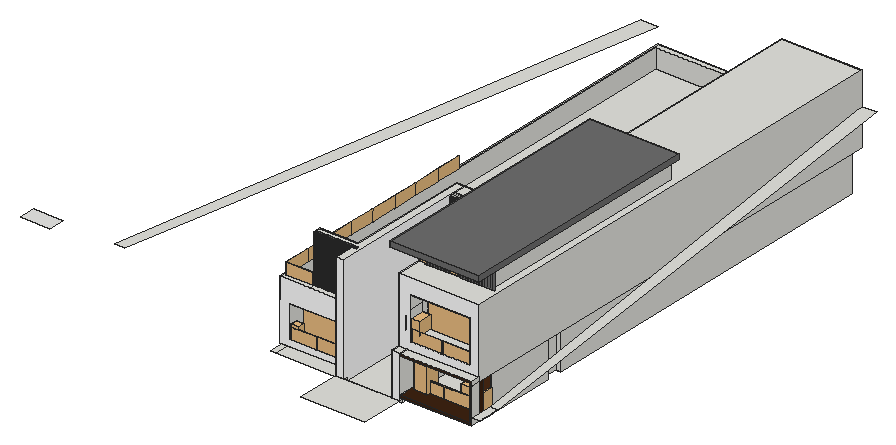
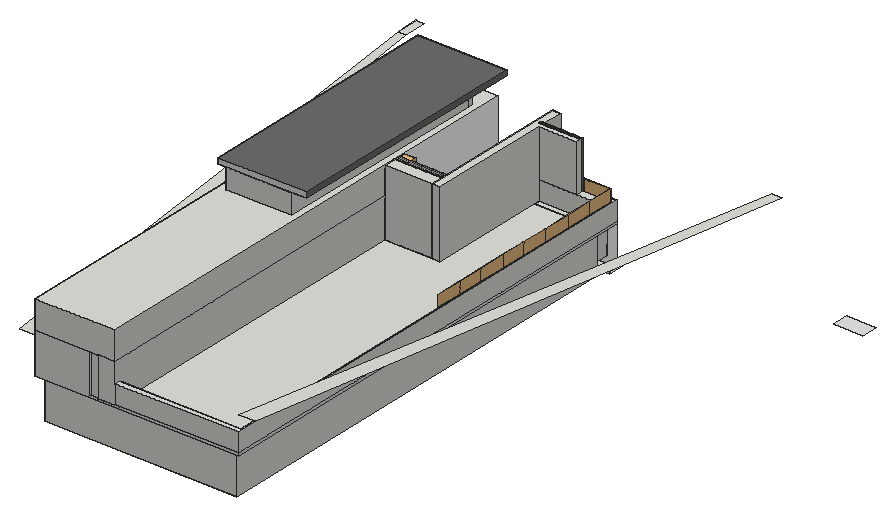
# SketchUp Ruby script. Lengths in inches.
U = 1.inch
M = Sketchup.active_model
def pt(a) = Geom::Point3d.new(a.map { |v| v * U })
def face(e, loops, mat)
  f = e.add_face(loops[0].map { |a| pt(a) })
  loops[1..].each { |l| e.add_face(l.map { |a| pt(a) }).erase! }
  f.material = f.back_material = mat if mat
  f
end
# faces: each face lists its corners as indices into pts; further lists are holes
def faces(e, pts, list, mat = nil) = list.each { |f| face(e, (f[0].is_a?(Array) ? f : [f]).map { |l| l.map { |i| pts[i] } }, mat) }
# xy, xz, yz: faces in a plane at the given z, y or x. An outline is a flat list of corners, or four numbers for a rectangle; further outlines are holes
def ring(l) = l.size == 4 ? [[l[0], l[1]], [l[2], l[1]], [l[2], l[3]], [l[0], l[3]]] : l.each_slice(2).to_a
def flat(e, list, mat, &to3) = list.each { |f| face(e, (f[0].is_a?(Array) ? f : [f]).map { |l| ring(l).map { |u, v| to3.(u, v) } }, mat) }
def xy(e, z, list, mat = nil) = flat(e, list, mat) { |x, y| [x, y, z] }
def xz(e, y, list, mat = nil) = flat(e, list, mat) { |x, z| [x, y, z] }
def yz(e, x, list, mat = nil) = flat(e, list, mat) { |y, z| [x, y, z] }
def lines(e, pts, list) = list.each { |a, b| e.add_line(pt(pts[a]), pt(pts[b])) }
# prism: a flat outline (further loops are holes) pulled along v
def prism(e, loops, v, mat = nil)
  f = face(e, loops, mat); d = Geom::Vector3d.new(v.map { |x| x * U })
  f.pushpull(f.normal.samedirection?(d) ? d.length : -d.length)
end
def box(e, o, s, mat = nil) = prism(e, [[o, [o[0] + s[0], o[1], o[2]], [o[0] + s[0], o[1] + s[1], o[2]], [o[0], o[1] + s[1], o[2]]]], [0, 0, s[2]], mat)
def at(x, y, z, deg = 0) = Geom::Transformation.translation(pt([x, y, z])) * Geom::Transformation.rotation(ORIGIN, Z_AXIS, deg.degrees)
def axes(o, x, y, z) = Geom::Transformation.new([*x, 0, *y, 0, *z, 0, *pt(o).to_a, 1])
def part(name) = M.definitions.add(name)
# library, detail: a bought-in or finely detailed component or shape, given as its bounding box
def library(name, o, s) = part(name).tap { |d| box(d.entities, o, s) }
def detail(e, o, s) = box(e.add_group.entities, o, s)
def put(e, d, t, mat = nil) = e.add_instance(d, t).tap { |i| i.material = mat if mat }
def group(e, t, mat = nil) = e.add_group.tap { |g| g.transformation = t; g.material = mat if mat }.entities
root = M.entities
M.materials.add("005").color = [231, 231, 229]
M.materials.add("[Color M00]").color = [255, 255, 255]
M.materials.add("[Color M04]").color = [109, 109, 109]
M.materials.add("[Color_F16]").color = [51, 102, 0]
M.materials.add("[Wood Cherry Original]1").color = [86, 49, 23]
M.materials.add("[Wood Veneer 01]").color = [61, 35, 18]
c1 = library("Obj_000003",[-31,-31.06,-7.89],[62,62.12,39.58])
c2 = library("Sliding Door",[0,0,0],[94.49,5.83,91.73])
c3 = library("plant1",[-367.84,-375.82,-125.45],[750.59,696.16,1346.74])
c4 = part("skp4FF")
put(c4.entities,c3,at(0,0,0))
c5 = library("Group5_1",[-7.56,-66.38,0.11],[6.33,135.04,120.95])
c6 = library("Group13",[-203.48,36.63,0],[29.68,67.31,50.64])
c7 = part("glass-railing")
detail(c7.entities,[0,0,0],[1.26,75.59,33.1875])
c8 = library("Foliage panel",[-0.08,0,0],[10.02,134.7,35.5])
c9 = library("Omni Light",[-12,-12,-12],[24,24,24])
c10 = library("Potted trailing plant",[-13.52,-13.75,-7.41],[40.56,40.5625,37.31])
c11 = part("Group\#1")
box(c11.entities,[0,-6.6875,0],[4.56,6.6875,139.36])
xy(root,160.97,[[958.48,680.42,1097.29,1084.23],[735.92,689.01,751.73,749.51],[751.73,689.01,934.66,749.51],[934.66,689.01,958.48,749.51],[1097.29,689.01,1121.6,749.51],
  [751.73,775.86,944.93,775.86,944.93,1121.05,1115.31,1121.05,1115.31,1027.76,1316.64,1027.76,1316.64,2093.94,751.73,2093.94],[1115.31,775.86,1307.58,775.86,1307.58,981.2,1299.77,981.2,1299.77,1027.76,1115.31,1027.76],[1307.58,775.86,1314.51,981.2]])
xy(root,167.65,[[735.92,723.48,934.66,749.51]])
xy(root,169.65,[[934.66,552.07,1121.6,680.42],[934.66,680.42,958.48,689.01],[1097.29,680.42,1121.6,689.01]])
xy(root,178.15,[[1121.6,680.42,1332.45,689.01],[1121.6,689.01,1326.45,706.73],[1326.45,689.01,1332.45,706.73],[1121.6,706.73,1326.45,745.61],[1121.6,745.61,1307.63,775.86]])
xy(root,184.15,[[1307.63,729.98,1326.45,745.61]])
xy(root,184.15,[[1121.6,680.42,1326.45,680.42,1326.45,729.98,1307.63,729.98,1307.63,745.61,1121.6,745.61]],"[Wood Veneer 01]")
xy(root,187.51,[[764.92,723.48,934.66,775.86]])
xy(root,253.22,[[0,691.02,86.73,739.27]],"005")
xy(root,280.97,[[764.92,723.48,934.66,775.86],[1307.58,775.86,1314.51,981.2],[1299.77,981.2,1316.64,1027.76],[944.93,1084.23,958.48,1121.05],[1097.29,1084.23,1115.31,1121.05]])
xy(root,280.97,[[[751.73,775.86,751.73,2093.94,1316.64,2093.94,1316.64,1027.76,1299.77,1027.76,1299.77,981.2,1307.58,981.2,1307.58,775.86,1115.31,775.86,1115.31,1121.05,944.93,1121.05,944.93,775.86],[1163.04,826.89,1164.08,827.02,1165.04,827.41,1165.875,828.05,1166.51,828.875,1166.91,829.84,1167.05,830.87,1166.92,831.91,1166.52,832.875,1165.89,833.7,1165.0625,834.34,1164.1,834.75,1163.07,834.89,1162.03,834.75,1161.0625,834.36,1160.23,833.72,1159.6,832.9,1159.19,831.93,1159.05,830.9,1159.1875,829.86,1159.58,828.9,1160.22,828.07,1161.04,827.43,1162.01,827.02],[1247.1,826.89,1248.14,827.02,1249.11,827.41,1249.9375,828.05,1250.57,828.875,1250.98,829.84,1251.12,830.87,1250.98,831.91,1250.59,832.875,1249.95,833.7,1249.125,834.34,1248.16,834.75,1247.13,834.89,1246.09,834.75,1245.125,834.36,1244.3,833.72,1243.66,832.9,1243.26,831.93,1243.12,830.9,1243.25,829.86,1243.65,828.9,1244.28,828.07,1245.11,827.43,1246.07,827.02]]],"[Color M00]")
xy(root,280.97,[[1121.6,729.98,1307.63,775.86]],"[Wood Cherry Original]1")
xy(root,282.4,[[1163.04,826.89,1162.01,827.02,1161.04,827.43,1160.22,828.07,1159.58,828.9,1159.1875,829.86,1159.05,830.9,1159.19,831.93,1159.6,832.9,1160.23,833.72,1161.0625,834.36,1162.03,834.75,1163.07,834.89,1164.1,834.75,1165.0625,834.34,1165.89,833.7,1166.52,832.875,1166.92,831.91,1167.05,830.87,1166.91,829.84,1166.51,828.875,1165.875,828.05,1165.04,827.41,1164.08,827.02],[1247.1,826.89,1246.07,827.02,1245.11,827.43,1244.28,828.07,1243.65,828.9,1243.25,829.86,1243.12,830.9,1243.26,831.93,1243.66,832.9,1244.3,833.72,1245.125,834.36,1246.09,834.75,1247.13,834.89,1248.16,834.75,1249.125,834.34,1249.95,833.7,1250.59,832.875,1250.98,831.91,1251.12,830.87,1250.98,829.84,1250.57,828.875,1249.9375,828.05,1249.11,827.41,1248.14,827.02]])
xy(root,286.97,[[741.77,759.55,764.92,759.55,764.92,775.86,934.66,775.86,934.66,1121.05,1097.29,1121.05,1097.29,2094.09,741.77,2094.09],[764.92,759.55,934.66,775.86],[1123.34,780.38,1317.15,780.38,1317.15,2083.7,1170.8,2083.7,1170.8,2109.75,1144.75,2109.75,1170.8,2108.5,1123.34,1119.8],[1123.34,1119.8,1097.29,1121.05,1097.29,2109.75,1144.75,2109.75,1170.8,2108.5]])
xy(root,287.46,[[1121.6,680.42,1326.45,729.98]],"[Wood Veneer 01]")
xy(root,293.34,[[1097.29,680.42,1121.6,706.73],[1121.6,680.42,1332.45,706.73]])
xy(root,316.52,[[1306.4375,706.73,1306.4375,780.38,1317.15,780.38]])
xy(root,316.72,[[1123.34,780.38,1304.94,1039.95]])
xy(root,317.41,[[1133.98,706.73,1306.4375,706.73,1306.4375,780.38,1123.34,780.38,1123.34,745.61,1133.98,745.61],[1121.36,745.61,1121.6,1119.8],[1121.6,745.61,1123.34,1119.8],[1123.34,780.38,1304.94,1039.95],[1304.94,780.38,1307.37,1039.95],
  [1307.37,780.38,1308.25,1039.95],[1308.25,780.38,1308.375,1039.95]])
xy(root,343.17,[[735.92,723.48,822.6,723.48,822.6,759.55,741.77,759.55,741.77,2094.09,1097.29,2094.09,1097.29,2109.75,735.92,2109.75],[822.6,723.48,934.66,745.61],[822.6,745.61,934.66,759.55]])
xy(root,388.75,[[1545.43,417,1566.68,482.75],[1566.68,417,1569.4,459.625],[1566.68,459.625,1569.4,459.625,1568.99,463.0625,1566.68,463.0625],[1569.4,459.625,1569.4,463.0625,1568.99,463.0625],[1566.68,463.0625,1568.99,463.0625,1566.68,482.75,1375.45,2109.75,1332.45,2109.75,1545.43,482.75,1566.68,482.75],
  [397.96,541.6875,426.77,541.6875,735.92,2109.75,685.89,2109.75]])
xy(root,400.97,[[1123.34,1119.8,1097.29,1121.05,1144.75,2109.75,1170.8,2108.5],[1170.8,2108.5,1144.75,2109.75,1170.8,2109.75]])
xy(root,441.33,[[1133.98,706.73,1133.98,745.61,1123.34,745.61,1123.34,1119.8,1170.8,2108.5,1170.8,2083.7,1317.15,2083.7,1317.15,780.38,1306.4375,780.38,1306.4375,706.73],[1121.36,745.61,1123.34,1119.8]])
xy(root,482.53,[[934.66,680.42,958.48,680.42,958.48,1121.05,934.66,1121.05,934.66,759.55,822.6,759.55,822.6,745.61,934.66,745.61],[958.48,1084.23,1097.29,1121.05]])
xy(root,484.15,[[[1097.29,706.73,1332.45,2109.75],[1115.6,791.02,1309.1,1438.15]]])
xy(root,543.9,[[1115.6,791.02,1309.1,1438.15]])
xy(root,543.9,[[[1072.18,706.73,1072.18,1438.15,1115.6,1438.15,1115.6,791.02,1309.1,791.02,1309.1,1438.15,1332.45,1438.15,1332.45,706.73],[1248.85,718.08,1250.23,718.26,1251.51,718.79,1252.61,719.64,1253.45,720.74,1253.99,722.02,1254.17,723.39,1253.99,724.77,1253.45,726.05,1252.61,727.15,1251.51,727.99,1250.23,728.52,1248.85,728.7,1247.48,728.52,1246.2,727.99,1245.1,727.15,1244.25,726.05,1243.72,724.77,1243.54,723.39,1243.72,722.02,1244.25,720.74,1245.1,719.64,1246.2,718.79,1247.48,718.26],[1160.21,719.39,1161.25,719.53,1162.21,719.93,1163.04,720.5625,1163.68,721.39,1164.08,722.36,1164.21,723.39,1164.08,724.43,1163.68,725.39,1163.04,726.22,1162.21,726.86,1161.25,727.26,1160.21,727.39,1159.18,727.26,1158.21,726.86,1157.39,726.22,1156.75,725.39,1156.35,724.43,1156.21,723.39,1156.35,722.36,1156.75,721.39,1157.39,720.5625,1158.21,719.93,1159.18,719.53]]],"[Color M04]")
xy(root,545.72,[[1248.85,718.08,1247.48,718.26,1246.2,718.79,1245.1,719.64,1244.25,720.74,1243.72,722.02,1243.54,723.39,1243.72,724.77,1244.25,726.05,1245.1,727.15,1246.2,727.99,1247.48,728.52,1248.85,728.7,1250.23,728.52,1251.51,727.99,1252.61,727.15,1253.45,726.05,1253.99,724.77,1254.17,723.39,1253.99,722.02,1253.45,720.74,1252.61,719.64,1251.51,718.79,1250.23,718.26],[1160.21,719.39,1159.18,719.53,1158.21,719.93,1157.39,720.5625,1156.75,721.39,1156.35,722.36,1156.21,723.39,1156.35,724.43,1156.75,725.39,1157.39,726.22,1158.21,726.86,1159.18,727.26,1160.21,727.39,1161.25,727.26,1162.21,726.86,1163.04,726.22,1163.68,725.39,1164.08,724.43,1164.21,723.39,1164.08,722.36,1163.68,721.39,1163.04,720.5625,1162.21,719.93,1161.25,719.53]],"[Color M04]")
xy(root,559.9,[[1072.18,706.73,1332.45,1438.15]],"[Color M04]")
xz(root,680.42,[[958.48,160.97,1097.29,169.65]])
xz(root,680.42,[[934.66,169.65,958.48,482.53],[1097.29,169.65,1121.6,293.34]],"[Color M00]")
xz(root,680.42,[[1121.6,178.15,1332.45,178.15,1332.45,293.34,1121.6,293.34,1121.6,287.46,1326.45,287.46,1326.45,184.15,1121.6,184.15]],"[Wood Veneer 01]")
xz(root,689.01,[[934.66,160.97,958.48,169.65],[1097.29,160.97,1121.6,169.65]])
xz(root,706.73,[[[1097.29,293.34,1332.45,484.15],[1133.98,317.41,1306.4375,441.33]]],"[Color M00]")
xz(root,706.73,[[1072.18,543.9,1332.45,559.9]],"[Color M04]")
xz(root,723.48,[[735.92,167.65,934.66,167.65,934.66,187.51,764.92,187.51,764.92,280.97,934.66,280.97,934.66,343.17,735.92,343.17]],"[Color M00]")
xz(root,729.98,[[1307.63,184.15,1326.45,184.15,1326.45,287.46,1121.6,287.46,1121.6,280.97,1307.63,280.97]],"[Wood Cherry Original]1")
xz(root,745.61,[[1121.6,178.15,1307.63,184.15],[1307.63,178.15,1326.45,184.15],[1121.36,317.41,1123.34,400.97],[1123.34,317.41,1133.98,400.97],[827.16,343.17,929.63,482.53],
  [929.63,343.17,934.66,482.53],[1121.36,400.97,1123.34,441.33],[1123.34,400.97,1133.98,441.33]])
xz(root,749.51,[[735.92,160.97,934.66,167.65]])
xz(root,759.55,[[741.77,286.97,934.66,343.17],[822.6,343.17,934.66,482.53]])
xz(root,775.86,[[751.73,160.97,751.73,183.39,764.92,183.39,764.92,187.51,934.66,187.51,934.66,280.97,944.93,280.97,944.93,160.97],[1115.31,160.97,1115.31,280.97,1121.6,280.97,1121.6,178.15,1307.58,178.15,1307.58,160.97],[1307.58,160.97,1307.58,178.15,1307.63,178.15,1307.63,280.97,1314.51,280.97,1314.51,160.97],[1307.58,178.15,1307.63,280.97],[751.73,183.39,764.92,280.97],
  [764.92,280.97,934.66,286.97]])
xz(root,780.38,[[1306.4375,316.52,1317.15,441.33],[1123.34,316.72,1304.94,317.41]])
xz(root,791.02,[[1122.35,484.15,1309.1,543.9]])
xz(root,981.2,[[1307.58,160.97,1314.51,280.97]])
xz(root,981.2,[[1299.77,160.97,1307.58,280.97]],"[Color M00]")
xz(root,1027.76,[[1299.77,160.97,1316.64,280.97]])
xz(root,1039.95,[[1123.34,316.72,1304.94,317.41]])
xz(root,1084.23,[[963.73,160.97,1097.29,482.53]])
xz(root,1119.8,[[1121.36,317.41,1123.34,441.33]])
xz(root,1121.05,[[944.93,160.97,1115.31,280.97],[958.48,280.97,1097.29,286.97],[934.66,286.97,958.48,482.53],[958.48,286.97,1097.29,482.53]])
xz(root,1438.15,[[1115.6,484.15,1309.1,543.9],[1072.18,543.9,1332.45,559.9]])
xz(root,2083.7,[[1170.8,286.97,1317.15,441.33]])
xz(root,2093.94,[[751.73,160.97,1316.64,280.97]])
xz(root,2094.09,[[741.77,286.97,1097.29,343.17]])
xz(root,2109.75,[[735.92,280.97,735.92,286.97,1170.8,286.97,1170.8,400.97,1332.45,400.97,1332.45,280.97],[735.92,286.97,1097.29,343.17],[1097.29,286.97,1144.75,400.97],[1097.29,400.97,1332.45,484.15]])
yz(root,735.92,[[723.48,280.97,2109.75,286.97],[723.48,286.97,2109.75,343.17]])
yz(root,741.77,[[759.55,286.97,2094.09,343.17]])
yz(root,751.73,[[775.86,160.97,2093.94,280.97]])
yz(root,764.92,[[723.48,187.51,775.86,280.97]])
yz(root,822.6,[[745.61,343.17,759.55,482.53]])
yz(root,934.66,[[689.01,160.97,689.01,169.65,680.42,169.65,680.42,280.97,775.86,280.97,775.86,187.51,723.48,187.51,723.48,167.65,749.51,167.65,749.51,160.97],[680.42,280.97,723.48,286.97],[723.48,280.97,775.86,286.97],[680.42,286.97,723.48,305.53],[723.48,286.97,759.55,343.17],
  [759.55,286.97,1121.05,482.53],[680.42,305.53,680.42,482.53,745.61,482.53,745.61,343.17,723.48,343.17,723.48,305.53]])
yz(root,944.93,[[775.86,160.97,1121.05,280.97]])
yz(root,958.48,[[680.42,160.97,689.01,169.65],[1084.23,280.97,1121.05,286.97],[1084.23,286.97,1121.05,482.53]])
yz(root,958.48,[[689.01,160.97,1084.23,160.97,1084.23,482.53,680.42,482.53,680.42,169.65,689.01,169.65]],"[Color M00]")
yz(root,1072.18,[[706.73,543.9,1438.15,559.9]],"[Color M04]")
yz(root,1097.29,[[680.42,160.97,689.01,169.65],[1084.23,280.97,1121.05,400.97],[1121.05,286.97,1121.05,400.97,2109.75,400.97,2109.75,343.17,2094.09,343.17,2094.09,286.97],[1084.23,400.97,1121.05,482.53],[1121.05,400.97,2109.75,484.15],
  [1084.23,482.53,1121.05,484.15]])
yz(root,1097.29,[[689.01,160.97,689.01,169.65,680.42,169.65,680.42,293.34,706.73,293.34,706.73,484.15,1084.23,484.15,1084.23,160.97]],"[Color M00]")
yz(root,1115.31,[[775.86,160.97,1121.05,280.97]])
yz(root,1115.6,[[791.02,484.15,1438.15,543.9]])
yz(root,1121.36,[[745.61,317.41,1119.8,400.97],[745.61,400.97,1119.8,441.33]])
yz(root,1121.6,[[680.42,169.65,689.01,178.15],[680.42,178.15,706.73,184.15],[745.61,178.15,775.86,178.15,775.86,280.97,729.98,280.97,729.98,287.46,680.42,287.46,680.42,184.15,745.61,184.15],[680.42,287.46,706.73,293.34],[706.73,287.46,745.61,293.34]])
yz(root,1123.34,[[780.38,286.97,1119.8,286.97,1119.8,317.41,1039.95,317.41,1039.95,316.72,780.38,316.72],[780.38,316.72,1039.95,317.41],[745.61,317.41,1119.8,400.97],[745.61,400.97,1119.8,441.33]])
yz(root,1133.98,[[706.73,317.41,745.61,400.97],[706.73,400.97,745.61,441.33]])
yz(root,1170.8,[[2083.7,286.97,2108.5,441.33],[2108.5,286.97,2109.75,400.97]])
yz(root,1299.77,[[981.2,160.97,1027.76,280.97]])
yz(root,1304.94,[[780.38,316.72,1039.95,317.41]])
yz(root,1306.4375,[[706.73,316.52,780.38,317.41],[706.73,317.41,780.38,441.33]])
yz(root,1307.58,[[775.86,160.97,981.2,280.97]],"[Wood Cherry Original]1")
yz(root,1307.63,[[745.61,178.15,745.61,184.15,729.98,184.15,729.98,280.97,775.86,280.97,775.86,178.15]],"[Wood Cherry Original]1")
yz(root,1309.1,[[791.02,484.15,1438.15,543.9]])
yz(root,1314.51,[[775.86,160.97,981.2,280.97]])
yz(root,1316.64,[[1027.76,160.97,2093.94,280.97]])
yz(root,1317.15,[[780.38,286.97,2083.7,441.33]])
yz(root,1326.45,[[706.73,178.15,745.61,184.15]])
yz(root,1326.45,[[680.42,184.15,729.98,287.46]],"[Wood Veneer 01]")
yz(root,1332.45,[[680.42,178.15,706.73,280.97],[680.42,280.97,706.73,293.34],[706.73,280.97,2109.75,484.15]])
yz(root,1332.45,[[706.73,543.9,1438.15,559.9]],"[Color M04]")
p = [[1163.04,826.89,280.97],[1162.01,827.02,280.97],[1162.01,827.02,282.4],[1163.04,826.89,282.4],[1164.08,827.02,280.97],[1164.08,827.02,282.4],
  [1247.1,826.89,280.97],[1246.07,827.02,280.97],[1246.07,827.02,282.4],[1247.1,826.89,282.4],[1248.14,827.02,280.97],[1248.14,827.02,282.4],
  [1161.04,827.43,280.97],[1161.04,827.43,282.4],[1165.04,827.41,280.97],[1165.04,827.41,282.4],[1245.11,827.43,280.97],[1245.11,827.43,282.4],
  [1249.11,827.41,280.97],[1249.11,827.41,282.4],[1160.22,828.07,280.97],[1160.22,828.07,282.4],[1165.875,828.05,280.97],[1165.875,828.05,282.4],
  [1244.28,828.07,280.97],[1244.28,828.07,282.4],[1249.9375,828.05,280.97],[1249.9375,828.05,282.4],[1166.51,828.875,280.97],[1166.51,828.875,282.4],
  [1250.57,828.875,280.97],[1250.57,828.875,282.4],[1159.58,828.9,280.97],[1159.58,828.9,282.4],[1243.65,828.9,280.97],[1243.65,828.9,282.4],
  [1159.1875,829.86,280.97],[1159.1875,829.86,282.4],[1166.91,829.84,280.97],[1166.91,829.84,282.4],[1243.25,829.86,280.97],[1243.25,829.86,282.4],
  [1250.98,829.84,280.97],[1250.98,829.84,282.4],[1167.05,830.87,280.97],[1167.05,830.87,282.4],[1251.12,830.87,280.97],[1251.12,830.87,282.4],
  [1159.05,830.9,280.97],[1159.05,830.9,282.4],[1243.12,830.9,280.97],[1243.12,830.9,282.4],[1159.19,831.93,280.97],[1159.19,831.93,282.4],
  [1166.92,831.91,280.97],[1166.92,831.91,282.4],[1243.26,831.93,280.97],[1243.26,831.93,282.4],[1250.98,831.91,280.97],[1250.98,831.91,282.4],
  [1159.6,832.9,280.97],[1159.6,832.9,282.4],[1166.52,832.875,280.97],[1166.52,832.875,282.4],[1243.66,832.9,280.97],[1243.66,832.9,282.4],
  [1250.59,832.875,280.97],[1250.59,832.875,282.4],[1160.23,833.72,280.97],[1160.23,833.72,282.4],[1165.89,833.7,280.97],[1165.89,833.7,282.4],
  [1244.3,833.72,280.97],[1244.3,833.72,282.4],[1249.95,833.7,280.97],[1249.95,833.7,282.4],[1161.0625,834.36,280.97],[1161.0625,834.36,282.4],
  [1165.0625,834.34,280.97],[1165.0625,834.34,282.4],[1245.125,834.36,280.97],[1245.125,834.36,282.4],[1249.125,834.34,280.97],[1249.125,834.34,282.4],
  [1164.1,834.75,280.97],[1164.1,834.75,282.4],[1248.16,834.75,280.97],[1248.16,834.75,282.4],[1162.03,834.75,280.97],[1162.03,834.75,282.4],
  [1246.09,834.75,280.97],[1246.09,834.75,282.4],[1163.07,834.89,280.97],[1163.07,834.89,282.4],[1247.13,834.89,280.97],[1247.13,834.89,282.4],
  [1097.29,1121.05,286.97],[1123.34,1119.8,286.97],[1123.34,1119.8,317.41],[1123.34,1119.8,400.97],[1097.29,1121.05,400.97],[1170.8,2108.5,286.97],
  [1170.8,2108.5,400.97],[1144.75,2109.75,286.97],[1144.75,2109.75,400.97],[1317.15,780.38,441.33],[1306.4375,706.73,441.33],[1306.4375,706.73,317.41],
  [1306.4375,706.73,316.52],[1317.15,780.38,316.52],[1170.8,2108.5,441.33],[1123.34,1119.8,441.33],[1248.85,718.08,543.9],[1247.48,718.26,543.9],
  [1247.48,718.26,545.72],[1248.85,718.08,545.72],[1250.23,718.26,543.9],[1250.23,718.26,545.72],[1246.2,718.79,543.9],[1246.2,718.79,545.72],
  [1251.51,718.79,543.9],[1251.51,718.79,545.72],[1245.1,719.64,543.9],[1245.1,719.64,545.72],[1252.61,719.64,543.9],[1252.61,719.64,545.72],
  [1160.21,719.39,543.9],[1159.18,719.53,543.9],[1159.18,719.53,545.72],[1160.21,719.39,545.72],[1161.25,719.53,543.9],[1161.25,719.53,545.72],
  [1158.21,719.93,543.9],[1158.21,719.93,545.72],[1162.21,719.93,543.9],[1162.21,719.93,545.72],[1244.25,720.74,543.9],[1244.25,720.74,545.72],
  [1253.45,720.74,543.9],[1253.45,720.74,545.72],[1157.39,720.5625,543.9],[1157.39,720.5625,545.72],[1163.04,720.5625,543.9],[1163.04,720.5625,545.72],
  [1156.75,721.39,543.9],[1156.75,721.39,545.72],[1163.68,721.39,543.9],[1163.68,721.39,545.72],[1243.72,722.02,543.9],[1243.72,722.02,545.72],
  [1253.99,722.02,543.9],[1253.99,722.02,545.72],[1156.35,722.36,543.9],[1156.35,722.36,545.72],[1164.08,722.36,543.9],[1164.08,722.36,545.72],
  [1243.54,723.39,543.9],[1243.54,723.39,545.72],[1254.17,723.39,543.9],[1254.17,723.39,545.72],[1156.21,723.39,543.9],[1156.21,723.39,545.72],
  [1164.21,723.39,543.9],[1164.21,723.39,545.72],[1156.35,724.43,543.9],[1156.35,724.43,545.72],[1164.08,724.43,543.9],[1164.08,724.43,545.72],
  [1243.72,724.77,543.9],[1243.72,724.77,545.72],[1253.99,724.77,543.9],[1253.99,724.77,545.72],[1156.75,725.39,543.9],[1156.75,725.39,545.72],
  [1163.68,725.39,543.9],[1163.68,725.39,545.72],[1244.25,726.05,543.9],[1244.25,726.05,545.72],[1253.45,726.05,543.9],[1253.45,726.05,545.72],
  [1157.39,726.22,543.9],[1157.39,726.22,545.72],[1163.04,726.22,543.9],[1163.04,726.22,545.72],[1245.1,727.15,543.9],[1245.1,727.15,545.72],
  [1252.61,727.15,543.9],[1252.61,727.15,545.72],[1158.21,726.86,543.9],[1158.21,726.86,545.72],[1162.21,726.86,543.9],[1162.21,726.86,545.72],
  [1159.18,727.26,543.9],[1159.18,727.26,545.72],[1161.25,727.26,543.9],[1161.25,727.26,545.72],[1246.2,727.99,543.9],[1246.2,727.99,545.72],
  [1251.51,727.99,543.9],[1251.51,727.99,545.72],[1160.21,727.39,543.9],[1160.21,727.39,545.72],[1247.48,728.52,543.9],[1247.48,728.52,545.72],
  [1250.23,728.52,543.9],[1250.23,728.52,545.72],[1248.85,728.7,543.9],[1248.85,728.7,545.72],[944.93,775.86,280.97],[958.48,775.86,280.97],
  [1115.31,775.86,280.97],[1097.29,775.86,280.97],[1308.375,1039.95,400.97],[1307.37,1039.95,400.97],[1121.36,745.61,441.33],[1121.36,706.73,441.33],
  [1121.36,745.61,400.97],[1121.36,706.73,400.97],[1123.34,745.61,441.33],[1123.34,706.73,441.33],[1316.64,1027.76,161.96],[1316.64,1021.76,160.97],
  [1308.375,780.38,400.97],[1308.25,780.38,400.97],[764.92,759.55,286.97],[764.92,745.61,286.97]]
faces(root,p,[[0,1,2,3],[4,0,3,5],[6,7,8,9],[10,6,9,11],[1,12,13,2],[14,4,5,15],[7,16,17,8],[18,10,11,19],
  [12,20,21,13],[22,14,15,23],[16,24,25,17],[26,18,19,27],[28,22,23,29],[30,26,27,31],[20,32,33,21],[24,34,35,25],
  [32,36,37,33],[38,28,29,39],[34,40,41,35],[42,30,31,43],[44,38,39,45],[46,42,43,47],[36,48,49,37],[40,50,51,41],
  [48,52,53,49],[54,44,45,55],[50,56,57,51],[58,46,47,59],[52,60,61,53],[62,54,55,63],[56,64,65,57],[66,58,59,67],
  [60,68,69,61],[70,62,63,71],[64,72,73,65],[74,66,67,75],[68,76,77,69],[78,70,71,79],[72,80,81,73],[82,74,75,83],
  [84,78,79,85],[86,82,83,87],[76,88,89,77],[80,90,91,81],[92,84,85,93],[94,86,87,95],[88,92,93,89],[90,94,95,91],
  [96,97,98,99,100],[98,97,101,102,99],[101,103,104,102],[105,106,107,108,109],[99,102,110,111]])
faces(root,p,[[112,113,114,115],[116,112,115,117],[113,118,119,114],[120,116,117,121],[118,122,123,119],[124,120,121,125],[126,127,128,129],[130,126,129,131],
  [127,132,133,128],[134,130,131,135],[122,136,137,123],[138,124,125,139],[132,140,141,133],[142,134,135,143],[140,144,145,141],[146,142,143,147],
  [136,148,149,137],[150,138,139,151],[144,152,153,145],[154,146,147,155],[148,156,157,149],[158,150,151,159],[152,160,161,153],[162,154,155,163],
  [160,164,165,161],[166,162,163,167],[156,168,169,157],[170,158,159,171],[164,172,173,165],[174,166,167,175],[168,176,177,169],[178,170,171,179],
  [172,180,181,173],[182,174,175,183],[176,184,185,177],[186,178,179,187],[180,188,189,181],[190,182,183,191],[188,192,193,189],[194,190,191,195],
  [184,196,197,185],[198,186,187,199],[192,200,201,193],[200,194,195,201],[196,202,203,197],[204,198,199,205],[202,206,207,203],[206,204,205,207]],"[Color M04]")
lines(root,p,[[208,209],[210,211],[212,213],[214,215],[216,217],[218,219],[220,221],[222,223],[224,225]])
put(root,c1,axes([1007.02,954,173.9],[0.94045,0.94045,-0.00073],[-1.09602,1.09602,0.00035],[0.0009,0.00038,1.64]),"[Color_F16]")
put(root,c2,axes([1115.31,979.97,160.97],[1.95222,0,0],[0,1,0],[0,0,1.30815]))
put(root,c4,axes([1076.94,1001.85,167.64],[0.05316,0,0],[0,0.05316,0],[0,0,0.05316]))
put(root,c4,axes([1048.81,1001.85,167.64],[0.05316,0,0],[0,0.05316,0],[0,0,0.05316]))
put(root,c4,axes([1020.63,1001.85,167.64],[0.05316,0,0],[0,0.05316,0],[0,0,0.05316]))
g1 = group(root,at(958.48,1084.23,160.97))
xy(g1,0,[[0,-16.875,5.26,0]])
xy(g1,321.5625,[[0,-16.875,5.26,0]])
xz(g1,-16.875,[[0,0,5.26,321.5625],[6,0,11.26,321.5625],[12,0,17.26,321.5625],[18,0,23.26,321.5625],[24,0,29.26,321.5625],
  [30,0,35.26,321.5625],[36,0,41.26,321.5625],[42,0,47.26,321.5625],[48,0,53.26,321.5625],[54,0,59.26,321.5625],
  [60,0,65.26,321.5625],[66,0,71.26,321.5625],[72,0,77.26,321.5625],[78,0,83.26,321.5625],[84,0,89.26,321.5625],
  [90,0,95.26,321.5625],[96,0,101.26,321.5625],[102,0,107.26,321.5625],[108,0,113.26,321.5625],[114,0,119.26,321.5625],
  [120,0,125.26,321.5625],[126,0,131.26,321.5625],[132.125,0,137.38,321.5625]],"[Color M04]")
xz(g1,0,[[0,0,5.26,321.5625]])
yz(g1,0,[[-16.875,0,0,120],[-16.875,120,0,126],[-16.875,126,0,321.5625]])
yz(g1,5.26,[[-16.875,0,0,321.5625]])
yz(g1,11.26,[[-16.875,0,0,321.5625]])
yz(g1,17.26,[[-16.875,0,0,321.5625]])
yz(g1,23.26,[[-16.875,0,0,321.5625]])
yz(g1,29.26,[[-16.875,0,0,321.5625]])
yz(g1,35.26,[[-16.875,0,0,321.5625]])
yz(g1,41.26,[[-16.875,0,0,321.5625]])
yz(g1,47.26,[[-16.875,0,0,321.5625]])
yz(g1,53.26,[[-16.875,0,0,321.5625]])
yz(g1,59.26,[[-16.875,0,0,321.5625]])
yz(g1,65.26,[[-16.875,0,0,321.5625]])
yz(g1,71.26,[[-16.875,0,0,321.5625]])
yz(g1,77.26,[[-16.875,0,0,321.5625]])
yz(g1,83.26,[[-16.875,0,0,321.5625]])
yz(g1,89.26,[[-16.875,0,0,321.5625]])
yz(g1,95.26,[[-16.875,0,0,321.5625]])
yz(g1,101.26,[[-16.875,0,0,321.5625]])
yz(g1,107.26,[[-16.875,0,0,321.5625]])
yz(g1,113.26,[[-16.875,0,0,321.5625]])
yz(g1,119.26,[[-16.875,0,0,321.5625]])
yz(g1,125.26,[[-16.875,0,0,321.5625]])
yz(g1,131.26,[[-16.875,0,0,321.5625]])
p = [[138.57,0,0],[138.57,0,321.5625],[137.38,-16.875,321.5625],[137.38,-16.875,0]]
faces(g1,p,[[0,1,2,3]])
put(root,c5,axes([1208.32,1009.07,163.54],[0,1.63,0],[1.33185,0,0],[0,0,0.97]))
put(root,c6,at(1351.34,949.66,178.15,90))
put(root,c7,axes([1308,729.52,184.15],[0,1,0],[-1.26151,0,0],[0,0,1]))
put(root,c7,axes([1212.67,729.52,184.15],[0,1,0],[-1.19536,0,0],[0,0,1]))
put(root,c4,axes([1148.53,741.9375,190.82],[0.05316,0,0],[0,0.05316,0],[0,0,0.05316]))
put(root,c2,axes([764.92,770.03,187.51],[1.79644,0,0],[0,1,0],[0,0,1.01875]))
put(root,c7,axes([935.61,723.4,187.51],[0,1,0],[-1.21,0,0],[0,0,1]))
put(root,c7,axes([844.16,722.85,187.51],[0,1,0],[-1.05,0,0],[0,0,1]))
put(root,c4,axes([917.74,734.65,191.24],[0.0297,0,0],[0,0.0297,0],[0,0,0.0297]))
put(root,c4,axes([778.12,734.65,191.24],[0.0297,0,0],[0,0.0297,0],[0,0,0.0297]))
put(root,c5,axes([848.36,774.63,187.95],[0,-1,0],[1.25699,0,0],[0,0,0.76837]))
put(root,c8,axes([993.98,1048.96,361.77],[0,1.85,0],[0,0,-1],[-1,0,0]))
put(root,c9,at(1162.03,834.75,278.65))
put(root,c9,at(1247.34,834.75,278.65))
put(root,c2,axes([1123.34,779.16,317.41],[1.93777,0,0],[0,1,0],[0,0,1.3509]))
put(root,c7,axes([1306.4375,706.73,317.41],[0,1,0],[-1.0769,0,0],[0,0,1]))
put(root,c7,axes([1225.08,706.73,317.41],[0,1,0],[-1.19536,0,0],[0,0,1]))
put(root,c5,axes([1213.14,782.78,321.04],[0,-1,0],[1.35288,0,0],[0,0,0.99]))
put(root,c10,at(1145.58,720.25,349.48,90))
put(root,c11,at(822.6,745.61,343.17),"[Color M04]")
put(root,c11,at(828.6,745.61,343.17),"[Color M04]")
put(root,c11,at(834.6,745.61,343.17),"[Color M04]")
put(root,c11,at(840.6,745.61,343.17),"[Color M04]")
put(root,c11,at(846.6,745.61,343.17),"[Color M04]")
put(root,c11,at(852.6,745.61,343.17),"[Color M04]")
put(root,c11,at(858.6,745.61,343.17),"[Color M04]")
put(root,c11,at(864.6,745.61,343.17),"[Color M04]")
put(root,c11,at(870.6,745.61,343.17),"[Color M04]")
put(root,c11,at(876.6,745.61,343.17),"[Color M04]")
put(root,c11,at(882.6,745.61,343.17),"[Color M04]")
put(root,c11,at(888.6,745.61,343.17),"[Color M04]")
put(root,c11,at(894.6,745.61,343.17),"[Color M04]")
put(root,c11,at(900.6,745.61,343.17),"[Color M04]")
put(root,c11,at(906.6,745.61,343.17),"[Color M04]")
put(root,c11,at(912.6,745.61,343.17),"[Color M04]")
put(root,c11,at(918.6,745.61,343.17),"[Color M04]")
put(root,c11,at(924.6,745.61,343.17),"[Color M04]")
put(root,c11,at(930.6,745.61,343.17),"[Color M04]")
put(root,c11,at(936.6,745.61,343.17),"[Color M04]")
put(root,c11,at(942.6,745.61,343.17),"[Color M04]")
put(root,c7,axes([821.6875,736.16,343.17],[0,1,0],[-1.05,0,0],[0,0,1]))
put(root,c7,axes([742.32,736.79,343.17],[1,0,0],[0,1.05,0],[0,0,1]))
put(root,c7,axes([742.32,816.16,343.17],[1,0,0],[0,1.05,0],[0,0,1]))
put(root,c7,axes([742.32,895.53,343.17],[1,0,0],[0,1.05,0],[0,0,1]))
put(root,c7,axes([742.32,974.9,343.17],[1,0,0],[0,1.05,0],[0,0,1]))
put(root,c7,axes([742.32,1054.27,343.17],[1,0,0],[0,1.05,0],[0,0,1]))
put(root,c7,axes([742.32,1132.81,343.17],[1,0,0],[0,1.05,0],[0,0,1]))
put(root,c7,axes([742.32,1212.18,343.17],[1,0,0],[0,1.05,0],[0,0,1]))
put(root,c7,axes([742.32,1290.23,343.17],[1,0,0],[0,1.05,0],[0,0,1]))
put(root,c8,axes([1061.78,1050.85,348.07],[0,1.85,0],[0,0,1],[1,0,0]))
g2 = group(root,at(1115.6,791.02,484.15))
xy(g2,0,[[0,-11.25,6.75,0]])
xy(g2,59.75,[[0,-11.25,6.75,0]])
xz(g2,-11.25,[[0,0,6.75,59.75],[8,0,14.75,59.75],[16,0,22.75,59.75],[24,0,30.75,59.75],[32,0,38.75,59.75],
  [40,0,46.75,59.75],[48,0,54.75,59.75],[56,0,62.75,59.75],[64,0,70.75,59.75],[72,0,78.75,59.75],
  [80,0,86.75,59.75],[88,0,94.75,59.75],[96,0,102.75,59.75],[104,0,110.75,59.75],[112,0,118.75,59.75],
  [120,0,126.75,59.75],[128,0,134.75,59.75],[136,0,142.75,59.75],[144,0,150.75,59.75],[152,0,158.75,59.75],
  [160,0,166.75,59.75],[167.5625,0,174.32,59.75],[175.125,0,181.88,59.75],[182.6875,0,189.44,59.75],[190.25,0,197,59.75],
  [197.8125,0,204.57,59.75]],"[Color M04]")
xz(g2,0,[[0,0,6.75,59.75]])
yz(g2,0,[[-11.25,0,0,59.75]])
yz(g2,6.75,[[-11.25,0,0,59.75]])
yz(g2,14.75,[[-11.25,0,0,59.75]])
yz(g2,22.75,[[-11.25,0,0,59.75]])
yz(g2,30.75,[[-11.25,0,0,59.75]])
yz(g2,38.75,[[-11.25,0,0,59.75]])
yz(g2,46.75,[[-11.25,0,0,59.75]])
yz(g2,54.75,[[-11.25,0,0,59.75]])
yz(g2,62.75,[[-11.25,0,0,59.75]])
yz(g2,70.75,[[-11.25,0,0,59.75]])
yz(g2,78.75,[[-11.25,0,0,59.75]])
yz(g2,86.75,[[-11.25,0,0,59.75]])
yz(g2,94.75,[[-11.25,0,0,59.75]])
yz(g2,102.75,[[-11.25,0,0,59.75]])
yz(g2,110.75,[[-11.25,0,0,59.75]])
yz(g2,118.75,[[-11.25,0,0,59.75]])
yz(g2,126.75,[[-11.25,0,0,59.75]])
yz(g2,134.75,[[-11.25,0,0,59.75]])
yz(g2,142.75,[[-11.25,0,0,59.75]])
yz(g2,150.75,[[-11.25,0,0,59.75]])
yz(g2,158.75,[[-11.25,0,0,59.75]])
yz(g2,166.75,[[-11.25,0,0,59.75]])
p = [[8,0,0],[8,-11.25,0],[8,0,59.75],[8,-11.25,59.75],[16,0,0],[16,-11.25,0],
  [16,0,59.75],[16,-11.25,59.75],[24,0,0],[24,-11.25,0],[24,0,59.75],[24,-11.25,59.75],
  [32,0,0],[32,-11.25,0],[32,0,59.75],[32,-11.25,59.75],[40,0,0],[40,-11.25,0],
  [40,0,59.75],[40,-11.25,59.75],[48,0,0],[48,-11.25,0],[48,0,59.75],[48,-11.25,59.75],
  [56,0,0],[56,-11.25,0],[56,0,59.75],[56,-11.25,59.75],[64,0,0],[64,-11.25,0],
  [64,0,59.75],[64,-11.25,59.75],[72,0,0],[72,-11.25,0],[72,0,59.75],[72,-11.25,59.75],
  [80,0,0],[80,-11.25,0],[80,0,59.75],[80,-11.25,59.75],[88,0,0],[88,-11.25,0],
  [88,0,59.75],[88,-11.25,59.75],[96,0,0],[96,-11.25,0],[96,0,59.75],[96,-11.25,59.75],
  [104,0,0],[104,-11.25,0],[104,0,59.75],[104,-11.25,59.75],[112,0,0],[112,-11.25,0],
  [112,0,59.75],[112,-11.25,59.75],[120,0,0],[120,-11.25,0],[120,0,59.75],[120,-11.25,59.75],
  [128,0,0],[128,-11.25,0],[128,0,59.75],[128,-11.25,59.75],[136,0,0],[136,-11.25,0],
  [136,0,59.75],[136,-11.25,59.75],[144,0,0],[144,-11.25,0],[144,0,59.75],[144,-11.25,59.75],
  [152,0,0],[152,-11.25,0],[152,0,59.75],[152,-11.25,59.75],[160,0,0],[160,-11.25,0],
  [160,0,59.75],[160,-11.25,59.75]]
lines(g2,p,[[0,1],[2,3],[4,5],[6,7],[8,9],[10,11],[12,13],[14,15],[16,17],[18,19],[20,21],[22,23],
  [24,25],[26,27],[28,29],[30,31],[32,33],[34,35],[36,37],[38,39],[40,41],[42,43],[44,45],[46,47],
  [48,49],[50,51],[52,53],[54,55],[56,57],[58,59],[60,61],[62,63],[64,65],[66,67],[68,69],[70,71],
  [72,73],[74,75],[76,77],[78,79]])
put(root,c9,axes([1251.51,727.99,543.9],[0,0,-1],[0,1,0],[1,0,0]))
put(root,c9,axes([1159.45,727.99,543.9],[0,0,-1],[0,1,0],[1,0,0]))
